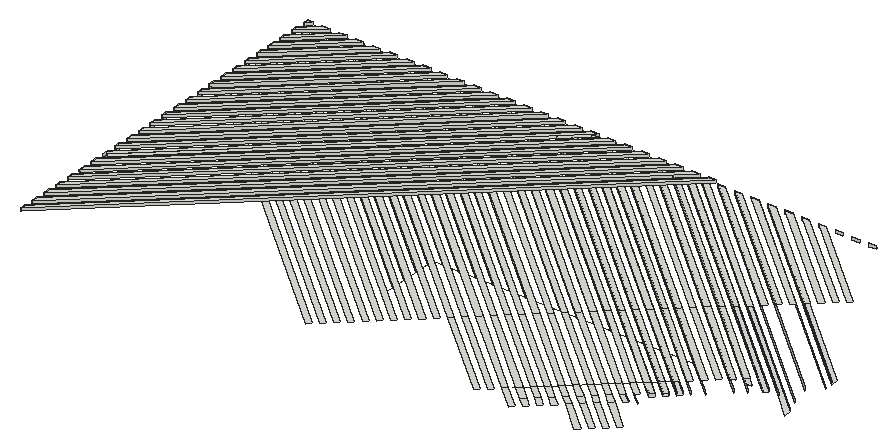
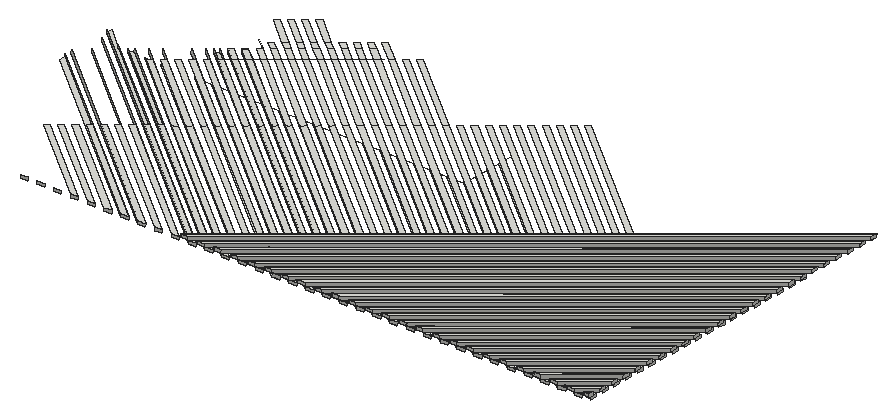
# SketchUp Ruby script. Lengths in inches.
U = 1.inch
M = Sketchup.active_model
def pt(a) = Geom::Point3d.new(a.map { |v| v * U })
def face(e, loops, mat)
  f = e.add_face(loops[0].map { |a| pt(a) })
  loops[1..].each { |l| e.add_face(l.map { |a| pt(a) }).erase! }
  f.material = f.back_material = mat if mat
  f
end
# faces: each face lists its corners as indices into pts; further lists are holes
def faces(e, pts, list, mat = nil) = list.each { |f| face(e, (f[0].is_a?(Array) ? f : [f]).map { |l| l.map { |i| pts[i] } }, mat) }
# xy, xz, yz: faces in a plane at the given z, y or x. An outline is a flat list of corners, or four numbers for a rectangle; further outlines are holes
def ring(l) = l.size == 4 ? [[l[0], l[1]], [l[2], l[1]], [l[2], l[3]], [l[0], l[3]]] : l.each_slice(2).to_a
def flat(e, list, mat, &to3) = list.each { |f| face(e, (f[0].is_a?(Array) ? f : [f]).map { |l| ring(l).map { |u, v| to3.(u, v) } }, mat) }
def xy(e, z, list, mat = nil) = flat(e, list, mat) { |x, y| [x, y, z] }
def xz(e, y, list, mat = nil) = flat(e, list, mat) { |x, z| [x, y, z] }
def yz(e, x, list, mat = nil) = flat(e, list, mat) { |y, z| [x, y, z] }
def lines(e, pts, list) = list.each { |a, b| e.add_line(pt(pts[a]), pt(pts[b])) }
# prism: a flat outline (further loops are holes) pulled along v
def prism(e, loops, v, mat = nil)
  f = face(e, loops, mat); d = Geom::Vector3d.new(v.map { |x| x * U })
  f.pushpull(f.normal.samedirection?(d) ? d.length : -d.length)
end
def box(e, o, s, mat = nil) = prism(e, [[o, [o[0] + s[0], o[1], o[2]], [o[0] + s[0], o[1] + s[1], o[2]], [o[0], o[1] + s[1], o[2]]]], [0, 0, s[2]], mat)
def at(x, y, z, deg = 0) = Geom::Transformation.translation(pt([x, y, z])) * Geom::Transformation.rotation(ORIGIN, Z_AXIS, deg.degrees)
def axes(o, x, y, z) = Geom::Transformation.new([*x, 0, *y, 0, *z, 0, *pt(o).to_a, 1])
def part(name) = M.definitions.add(name)
# library, detail: a bought-in or finely detailed component or shape, given as its bounding box
def library(name, o, s) = part(name).tap { |d| box(d.entities, o, s) }
def detail(e, o, s) = box(e.add_group.entities, o, s)
def put(e, d, t, mat = nil) = e.add_instance(d, t).tap { |i| i.material = mat if mat }
def group(e, t, mat = nil) = e.add_group.tap { |g| g.transformation = t; g.material = mat if mat }.entities
root = M.entities
yz(root,1643.753,[[641.527,112.68,643.815,112.761,643.793,113.788,641.504,113.707]])
yz(root,1643.781,[[646.852,112.869,646.829,113.896,649.182,113.979,649.205,112.952]])
yz(root,1643.818,[[650.825,111.952,650.802,112.979,653.091,113.06,653.113,112.033]])
yz(root,1643.819,[[640.161,111.574,640.139,112.601,642.427,112.682,642.45,111.655],[645.46,111.762,645.437,112.789,647.79,112.872,647.813,111.845]])
yz(root,1643.82,[[624.133,111.006,624.11,112.033,626.463,112.116,626.486,111.089],[629.498,111.196,629.475,112.223,631.764,112.304,631.786,111.277]])
yz(root,1643.821,[[613.469,110.628,613.447,111.655,615.8,111.738,615.822,110.711],[618.834,110.818,618.812,111.845,621.1,111.926,621.123,110.899]])
yz(root,1643.822,[[602.806,110.25,602.783,111.277,605.136,111.36,605.159,110.333],[608.171,110.44,608.148,111.467,610.437,111.548,610.459,110.521]])
yz(root,1643.823,[[586.844,109.684,589.132,109.765,589.11,110.792,586.821,110.711],[592.143,109.872,594.496,109.955,594.473,110.982,592.12,110.899]])
yz(root,1643.824,[[576.181,109.306,578.469,109.387,578.446,110.414,576.158,110.333],[581.479,109.494,583.832,109.577,583.81,110.604,581.456,110.521]])
yz(root,1643.825,[[560.152,108.738,562.505,108.821,562.483,109.848,560.13,109.765],[565.517,108.928,567.806,109.009,567.783,110.036,565.494,109.955]])
yz(root,1643.826,[[554.854,108.55,557.142,108.631,557.119,109.658,554.831,109.577]])
p = [[1824.097,523.211,108.456],[1816.22,530.052,108.698],[1814.866,528.875,108.657],[1822.742,522.034,108.414],[1824.886,573.509,109.211],[1850.385,551.364,108.426],
  [1850.385,551.341,109.453],[1845.556,555.535,109.602],[1814.866,582.188,110.547],[1732.252,653.937,113.09],[1732.252,653.96,112.063],[1851.739,552.54,108.468],
  [1851.739,552.518,109.495],[1827.595,573.509,109.211],[1643.821,613.447,111.655],[1747.351,523.533,108.467],[1748.706,524.71,108.509],[1645.435,614.399,111.689],
  [1645.176,614.623,111.697],[1643.821,615.8,111.738],[1778.04,550.195,109.412],[1808.727,523.543,108.468],[1810.082,524.72,108.509],[1779.394,551.371,109.454],
  [1845.566,523.538,108.467],[1846.92,524.715,108.509],[1836.372,533.876,108.834],[1835.018,532.699,108.792],[1643.135,523.684,108.502],[1643.147,525.983,108.584],
  [1643.137,523.686,108.502],[1643.137,523.663,109.529],[1643.147,525.96,109.611],[1643.151,523.675,109.53],[1643.151,523.697,108.503],[1793.076,653.94,113.12],
  [1793.076,653.917,114.147],[1643.162,525.996,108.584],[1790.442,653.94,113.12],[1825.83,524.717,108.509],[1827.147,525.861,108.55],[1824.1,528.508,108.644],
  [1822.783,527.363,108.603],[1734.961,653.96,112.063],[1734.961,653.937,113.09],[1816.22,583.365,110.588],[1846.91,556.711,109.643],[1831.0625,573.509,109.211],
  [1853.473,554.046,108.521],[1853.473,554.024,109.548],[1848.644,558.217,109.697],[1817.954,584.871,110.642],[1738.428,653.9375,113.09],[1738.428,653.96,112.063],
  [1833.697,573.509,109.211],[1854.79,555.191,108.562],[1643.149,525.962,109.611],[1643.162,525.974,109.611],[1790.442,653.917,114.147],[1643.821,618.812,111.845],
  [1750.439,526.216,108.562],[1751.757,527.36,108.603],[1645.138,619.956,111.886],[1643.821,621.1,111.926],[1781.128,552.877,109.507],[1811.816,526.226,108.5625],
  [1813.133,527.37,108.603],[1782.445,554.022,109.548],[1848.654,526.221,108.5625],[1849.971,527.365,108.603],[1839.423,536.526,108.928],[1838.106,535.382,108.887],
  [1819.271,532.702,108.792],[1817.954,531.558,108.752],[1828.88,527.367,108.603],[1830.234,528.543,108.645],[1827.1875,531.189,108.739],[1825.833,530.013,108.697],
  [1753.929,555.196,108.562],[1643.818,650.825,111.952],[1643.818,653.113,112.033],[1645.136,651.969,111.993],[1649.024,648.592,111.873],[1753.929,557.485,108.643],
  [1741.0625,653.96,112.063],[1741.0625,653.9375,113.09],[1819.271,586.015,110.682],[1849.961,559.362,109.737],[1854.79,555.168,109.589],[1837.162,573.51,109.211],
  [1856.523,556.696,108.615],[1856.523,556.673,109.642],[1851.694,560.867,109.791],[1821.004,587.521,110.736],[1744.528,653.938,113.09],[1744.528,653.96,112.063],
  [1839.871,573.51,109.211],[1857.877,557.872,108.657],[1643.82,624.11,112.033],[1753.489,528.866,108.656],[1754.844,530.042,108.698],[1648.824,622.117,111.962],
  [1645.175,625.287,112.075],[1643.82,626.463,112.116],[1784.178,555.527,109.601],[1785.532,556.704,109.643],[1842.51,539.208,109.023],[1841.155,538.031,108.981],
  [1851.703,528.871,108.656],[1853.057,530.048,108.698],[1643.162,529.008,108.691],[1643.175,531.372,108.775],[1643.165,529.011,108.691],[1643.165,528.988,109.718],
  [1643.175,531.349,109.802],[1643.19,531.385,108.775],[1643.178,529.022,108.691],[1786.974,653.94,113.12],[1784.265,653.94,113.12],[1643.178,528.999,109.718],
  [1786.974,653.917,114.147],[1822.358,535.384,108.887],[1821.004,534.207,108.846],[1831.968,530.049,108.698],[1833.285,531.194,108.739],[1830.238,533.84,108.833],
  [1828.921,532.695,108.792],[1747.237,653.961,112.063],[1747.237,653.938,113.09],[1822.358,588.697,110.777],[1853.048,562.043,109.832],[1857.877,557.85,109.684],
  [1843.339,573.51,109.211],[1859.611,559.379,108.71],[1859.611,559.356,109.737],[1854.782,563.549,109.886],[1824.092,590.203,110.831],[1750.705,653.938,113.09],
  [1750.705,653.961,112.063],[1650.66,650.181,111.929],[1646.315,653.955,112.063],[1649.024,653.955,112.063],[1753.928,562.848,108.833],[1753.928,560.495,108.75],
  [1643.177,531.352,109.802],[1643.19,531.363,109.802],[1784.265,653.917,114.147],[1643.82,629.475,112.223],[1756.577,531.548,108.751],[1757.894,532.693,108.792],
  [1645.849,630.001,112.242],[1645.137,630.619,112.264],[1643.82,631.764,112.304],[1787.266,558.21,109.697],[1788.583,559.354,109.737],[1845.561,541.858,109.117],
  [1844.243,540.714,109.076],[1854.791,531.554,108.752],[1856.108,532.698,108.792],[1825.409,538.034,108.981],[1824.092,536.89,108.941],[1833.325,536.522,108.928],
  [1831.971,535.345,108.886],[1643.82,634.774,112.411],[1759.627,534.198,108.845],[1760.981,535.374,108.887],[1648.863,632.746,112.339],[1645.174,635.95,112.453],
  [1643.819,637.127,112.494],[1790.315,560.859,109.79],[1791.67,562.036,109.832],[1849.439,573.51,109.211],[1862.66,562.028,108.804],[1862.66,562.005,109.831],
  [1857.832,566.199,109.98],[1827.141,592.853,110.925],[1756.805,653.939,113.09],[1756.805,653.961,112.063],[1643.19,534.396,108.882],[1643.202,536.695,108.963],
  [1643.193,534.399,108.882],[1643.217,536.708,108.964],[1643.205,534.409,108.882],[1780.8,653.939,113.12],[1778.165,653.939,113.12],[1643.193,534.376,109.909],
  [1643.202,536.672,109.99],[1643.205,534.386,109.909],[1780.8,653.917,114.147],[1828.496,540.716,109.076],[1827.142,539.539,109.035],[1836.376,539.172,109.022],
  [1835.059,538.028,108.981],[1643.819,640.139,112.601],[1762.715,536.881,108.94],[1764.032,538.025,108.981],[1648.646,638.235,112.534],[1645.905,640.615,112.618],
  [1645.136,641.283,112.642],[1643.819,642.427,112.682],[1793.403,563.542,109.886],[1794.72,564.686,109.926],[1656.638,650.354,111.936],[1652.491,653.955,112.063],
  [1655.126,653.955,112.063],[1753.928,568.148,109.021],[1753.928,565.86,108.94],[1643.205,536.675,109.99],[1643.217,536.685,109.991],[1778.165,653.917,114.147],
  [1831.547,543.366,109.17],[1830.23,542.222,109.13],[1839.463,541.854,109.117],[1838.109,540.677,109.075],[1643.819,645.437,112.789],[1765.765,539.53,109.034],
  [1767.119,540.707,109.076],[1648.501,643.723,112.728],[1645.173,646.614,112.831],[1643.819,647.79,112.872],[1796.453,566.191,109.98],[1797.807,567.368,110.021],
  [1790.169,653.963,112.064],[1888.287,568.751,109.043],[1888.287,566.462,108.961],[1880.169,573.512,109.211],[1787.535,653.963,112.064],[1861.716,573.511,109.211],
  [1868.798,567.36,108.993],[1868.798,567.337,110.02],[1863.97,571.531,110.169],[1833.279,598.185,111.114],[1769.081,653.939,113.09],[1769.081,653.962,112.063],
  [1843.822,607.345,111.438],[1882.387,573.852,110.251],[1888.287,568.728,110.069],[1790.169,653.941,113.09],[1643.218,539.72,109.071],[1643.23,542.084,109.155],
  [1643.221,539.723,109.071],[1643.245,542.097,109.155],[1643.233,539.733,109.071],[1643.221,539.701,110.098],[1643.23,542.062,110.181],[1643.233,539.711,110.098],
  [1774.697,653.939,113.12],[1774.697,653.916,114.147],[1771.988,653.939,113.12],[1834.634,546.048,109.265],[1833.28,544.871,109.224],[1842.514,544.504,109.211],
  [1841.197,543.36,109.17],[1647.158,647.902,112.876],[1768.852,542.213,109.129],[1770.17,543.357,109.17],[1648.693,648.857,112.91],[1645.136,651.946,113.02],
  [1643.818,653.091,113.06],[1643.818,650.802,112.979],[1799.541,568.874,110.075],[1800.858,570.019,110.115],[1867.892,573.512,109.211],[1871.886,570.043,109.088],
  [1871.886,570.02,110.115],[1867.058,574.213,110.264],[1836.367,600.868,111.209],[1775.258,653.94,113.09],[1775.258,653.962,112.063],[1643.824,573.146,110.226],
  [1643.825,570.793,110.143],[1643.825,570.816,109.116],[1643.824,573.169,109.199],[1666.086,647.447,111.832],[1658.592,653.955,112.063],[1661.301,653.955,112.063],
  [1753.935,573.505,109.211],[1753.927,573.505,109.211],[1753.927,571.158,109.128],[1643.233,542.065,110.182],[1643.245,542.074,110.182],[1771.988,653.916,114.147],
  [1837.685,548.698,109.359],[1836.368,547.554,109.319],[1847.293,543.363,109.17],[1848.646,544.539,109.212],[1845.601,547.186,109.306],[1844.247,546.009,109.264],
  [1848.647,544.54,109.212],[1650.696,650.127,112.955],[1771.902,544.862,109.223],[1773.257,546.039,109.265],[1649.024,653.932,113.09],[1646.315,653.932,113.09],
  [1802.591,571.524,110.169],[1803.945,572.7,110.21],[1873.992,573.512,109.211],[1874.936,572.692,109.182],[1874.936,572.67,110.209],[1870.108,576.863,110.358],
  [1839.417,603.517,111.303],[1781.358,653.94,113.09],[1781.358,653.963,112.064],[1784.067,653.963,112.064],[1876.291,573.869,109.224],[1875.88,573.512,109.211],
  [1672.223,647.481,111.834],[1664.768,653.956,112.063],[1667.403,653.956,112.063],[1760.037,573.505,109.211],[1757.402,573.505,109.211],[1675.176,650.215,111.931],
  [1670.868,653.956,112.063],[1673.577,653.956,112.063],[1766.212,573.505,109.211],[1763.503,573.505,109.211],[1681.352,650.216,111.931],[1677.045,653.956,112.063],
  [1679.679,653.957,112.063],[1772.314,573.506,109.211],[1769.679,573.506,109.211],[1688.123,649.634,111.91],[1683.145,653.957,112.063],[1685.854,653.957,112.063],
  [1778.488,573.506,109.211],[1775.779,573.506,109.211],[1694.299,649.634,111.91],[1689.321,653.957,112.063],[1691.956,653.957,112.063],[1784.59,573.507,109.211],
  [1781.956,573.506,109.211],[1700.724,649.352,111.9],[1695.422,653.958,112.063],[1698.131,653.958,112.063],[1790.765,573.507,109.211],[1788.056,573.507,109.211],
  [1806.509,573.508,109.211],[1713.875,653.959,112.063],[1716.509,653.959,112.063],[1809.144,573.508,109.211],[1812.609,573.508,109.211],[1719.975,653.959,112.063],
  [1722.684,653.959,112.063],[1815.318,573.508,109.211],[1818.786,573.509,109.211],[1726.151,653.959,112.063],[1728.786,653.959,112.063],[1821.42,573.509,109.211],
  [1753.339,653.961,112.063],[1845.974,573.51,109.211],[1759.514,653.961,112.063],[1852.148,573.511,109.211],[1771.79,653.962,112.063],[1864.425,573.511,109.211],
  [1777.893,653.962,112.063],[1870.527,573.512,109.211],[1880.169,573.49,110.238],[1842.505,606.2,111.398],[1787.535,653.94,113.09],[1793.635,653.963,112.064],
  [1886.269,573.513,109.211],[1886.269,573.49,110.238],[1884.119,575.357,110.304],[1845.554,608.85,111.492],[1793.635,653.941,113.09],[1784.067,653.94,113.09],
  [1840.771,604.694,111.345],[1871.463,578.039,110.4],[1876.291,573.846,110.251],[1848.608,547.519,109.347],[1851.662,544.872,109.253],[1851.658,544.868,109.253],
  [1848.607,547.518,109.347],[1653.992,554.422,110.62],[1643.26,545.098,110.289],[1643.249,545.089,110.289],[1643.249,545.111,109.262],[1643.26,545.121,109.262],
  [1649.213,550.292,109.446],[1768.523,653.939,113.12],[1768.523,653.916,114.147],[1643.257,547.384,110.37],[1643.257,547.407,109.343],[1643.272,547.42,109.344],
  [1647.895,551.436,109.486],[1840.772,551.379,109.454],[1839.418,550.203,109.413],[1649.742,553.04,109.543],[1643.261,547.388,110.37],[1643.272,547.397,110.371],
  [1652.935,555.791,110.668],[1765.888,653.916,114.147],[1765.888,653.938,113.12],[1656.638,650.331,112.962],[1774.99,547.545,109.318],[1776.307,548.689,109.359],
  [1655.126,653.933,113.09],[1652.491,653.932,113.09],[1847.252,548.695,109.389],[1805.679,574.206,110.264],[1806.996,575.351,110.304],[1848.652,549.836,109.4],
  [1843.823,554.03,109.548],[1842.506,552.885,109.508],[1847.335,548.692,109.359],[1665.424,647.999,112.88],[1661.301,653.933,113.09],[1658.592,653.933,113.09],
  [1808.728,576.856,110.358],[1810.083,578.033,110.399],[1648.834,555.241,110.649],[1643.287,550.422,110.478],[1643.277,550.414,110.478],[1643.277,550.436,109.451],
  [1643.287,550.445,109.451],[1646.161,552.942,109.539],[1650.485,556.698,109.673],[1762.421,653.938,113.12],[1762.421,653.916,114.147],[1643.273,550.432,109.451],
  [1643.285,552.796,109.534],[1643.299,552.809,109.535],[1643.285,552.774,110.561],[1644.807,554.118,109.581],[1646.715,555.776,109.64],[1643.289,552.778,110.561],
  [1643.299,552.786,110.562],[1646.387,555.469,110.657],[1759.712,653.915,114.147],[1759.712,653.938,113.12],[1671.6,648,112.88],[1667.403,653.933,113.09],
  [1664.768,653.933,113.09],[1811.816,579.539,110.453],[1813.133,580.683,110.493],[1881.944,582.633,109.535],[1884.162,580.707,109.466],[1884.162,580.684,110.493],
  [1848.642,611.532,111.587],[1799.811,653.941,113.09],[1799.811,653.964,112.064],[1675.176,650.193,112.958],[1673.577,653.934,113.09],[1670.868,653.933,113.09],
  [1643.3,555.82,109.642],[1643.312,558.119,109.723],[1643.305,555.824,109.642],[1643.326,558.131,109.723],[1643.315,555.832,109.642],[1756.246,653.915,114.147],
  [1643.315,555.81,110.669],[1643.305,555.802,110.669],[1756.246,653.938,113.12],[1643.312,558.096,110.75],[1753.612,653.938,113.12],[1853.046,615.359,111.723],
  [1888.285,584.754,110.638],[1888.285,584.777,109.611],[1808.62,653.964,112.064],[1808.62,653.942,113.09],[1643.317,558.101,110.75],[1643.326,558.109,110.75],
  [1753.612,653.915,114.147],[1683.983,647.908,112.877],[1679.679,653.934,113.09],[1677.045,653.934,113.09],[1888.285,587.789,109.717],[1812.088,653.964,112.064],
  [1814.723,653.965,112.064],[1888.285,590.077,109.799],[1888.285,587.766,110.744],[1854.78,616.865,111.776],[1812.088,653.942,113.09],[1690.639,647.425,112.859],
  [1685.854,653.934,113.09],[1683.145,653.934,113.09],[1643.34,563.508,109.914],[1643.345,563.513,109.914],[1643.328,561.144,109.83],[1643.345,563.49,110.941],
  [1643.328,561.122,110.857],[1643.354,563.52,109.915],[1643.342,561.157,109.831],[1750.144,653.9375,113.12],[1747.435,653.9375,113.12],[1747.435,653.915,114.147],
  [1643.354,563.498,110.941],[1693.825,650.023,112.952],[1691.956,653.935,113.09],[1689.321,653.935,113.09],[1856.099,564.694,109.926],[1825.409,591.348,110.871],
  [1699.728,650.195,112.958],[1698.131,653.935,113.09],[1695.422,653.935,113.09],[1859.187,567.375,110.021],[1828.496,594.03,110.966],[1643.355,566.532,110.021],
  [1643.367,568.831,110.103],[1643.361,566.537,110.021],[1643.381,568.843,110.103],[1643.369,566.544,110.022],[1743.97,653.937,113.12],[1741.335,653.937,113.12],
  [1643.369,566.522,111.049],[1643.361,566.514,111.048],[1743.97,653.915,114.147],[1643.367,568.808,111.13],[1643.373,568.813,111.13],[1643.381,568.82,111.13],
  [1741.335,653.914,114.147],[1705.637,650.428,112.966],[1704.233,653.935,113.09],[1701.598,653.935,113.09],[1830.229,595.536,111.02],[1860.92,568.881,110.075],
  [1862.237,570.026,110.115],[1831.547,596.68,111.06],[1643.823,597.485,111.089],[1643.822,599.773,111.17],[1643.822,599.796,110.143],[1643.823,597.507,110.062],
  [1707.698,653.936,113.09],[1710.407,653.936,113.09],[1865.325,572.707,110.211],[1834.633,599.362,111.155],[1643.397,571.846,111.237],[1643.389,571.839,111.237],
  [1643.389,571.862,110.21],[1643.397,571.868,110.21],[1737.867,653.937,113.12],[1737.867,653.914,114.147],[1643.395,574.198,111.321],[1643.395,574.22,110.294],
  [1643.383,571.857,110.21],[1643.409,574.232,110.294],[1735.158,653.937,113.12],[1643.822,602.806,110.25],[1643.822,605.159,110.333],[1645.177,603.983,110.292],
  [1643.401,574.203,111.321],[1643.409,574.21,111.321],[1735.158,653.914,114.147],[1713.875,653.936,113.09],[1716.509,653.936,113.09],[1868.376,575.358,110.304],
  [1837.684,602.012,111.249],[1643.822,605.136,111.36],[1645.177,603.96,111.319],[1719.975,653.936,113.09],[1722.684,653.937,113.09],[1643.411,577.244,110.401],
  [1643.422,579.543,110.483],[1643.417,577.25,110.401],[1643.424,577.233,111.428],[1643.417,577.227,111.428],[1643.424,577.256,110.401],[1731.693,653.936,113.12],
  [1731.693,653.914,114.147],[1643.422,579.52,111.509],[1643.436,579.555,110.483],[1729.058,653.936,113.12],[1643.822,608.171,110.44],[1643.822,610.459,110.521],
  [1645.139,609.315,110.481],[1643.429,579.526,111.51],[1643.436,579.532,111.51],[1729.058,653.914,114.147],[1726.151,653.937,113.09],[1728.786,653.937,113.09],
  [1643.822,610.437,111.548],[1645.139,609.293,111.508],[1643.438,582.569,110.59],[1643.45,584.932,110.674],[1643.445,582.575,110.59],[1643.451,582.558,111.617],
  [1643.445,582.552,111.617],[1643.451,582.58,110.59],[1725.591,653.936,113.12],[1725.591,653.913,114.147],[1643.45,584.91,111.701],[1643.463,584.944,110.674],
  [1722.882,653.936,113.12],[1643.821,613.469,110.628],[1643.821,615.822,110.711],[1645.176,614.646,110.67],[1643.457,584.916,111.701],[1643.463,584.921,111.701],
  [1722.882,653.913,114.147],[1643.479,587.945,111.808],[1643.473,587.94,111.808],[1643.473,587.963,110.781],[1643.479,587.968,110.781],[1719.416,653.936,113.12],
  [1719.416,653.913,114.147],[1643.478,590.232,111.889],[1643.478,590.255,110.862],[1643.466,587.956,110.781],[1643.491,590.266,110.863],[1716.782,653.936,113.12],
  [1753.339,653.938,113.09],[1643.821,618.834,110.818],[1643.821,621.123,110.899],[1645.138,619.979,110.859],[1643.333,561.126,110.857],[1643.342,561.134,110.858],
  [1750.144,653.915,114.147],[1643.485,590.239,111.889],[1643.491,590.244,111.89],[1716.782,653.913,114.147],[1759.514,653.939,113.09],[1705.723,647.341,112.886],
  [1643.506,593.292,110.97],[1643.518,595.656,111.054],[1702.045,646.499,112.856],[1704.368,648.517,112.928],[1643.505,595.622,112.08],[1643.505,595.644,111.053],
  [1643.501,593.288,110.97],[1643.501,593.265,111.997],[1643.506,593.269,111.997],[1713.314,653.935,113.12],[1713.314,653.913,114.147],[1701.477,643.63,113.782],
  [1643.493,593.281,110.97],[1762.981,653.939,113.09],[1765.616,653.939,113.09],[1643.82,624.133,111.006],[1643.82,626.486,111.089],[1645.175,625.309,111.048],
  [1643.513,595.629,112.081],[1643.518,595.633,112.081],[1710.605,653.913,114.147],[1710.605,653.935,113.12],[1771.79,653.939,113.09],[1643.533,598.657,112.188],
  [1643.529,598.653,112.188],[1643.529,598.676,111.161],[1643.533,598.679,111.161],[1707.14,653.935,113.12],[1707.14,653.912,114.147],[1703.361,650.63,114.03],
  [1643.533,600.967,111.242],[1643.545,600.978,111.242],[1643.533,600.945,112.269],[1704.505,653.935,113.12],[1643.541,600.952,112.269],[1643.545,600.955,112.269],
  [1704.505,653.912,114.147],[1777.893,653.94,113.09],[1643.82,629.498,111.196],[1643.82,631.786,111.277],[1645.137,630.642,111.237],[1643.548,603.993,111.349],
  [1643.56,606.357,111.433],[1643.557,604,111.35],[1643.561,603.981,112.377],[1643.557,603.978,112.377],[1643.561,604.004,111.35],[1701.038,653.935,113.12],
  [1701.038,653.912,114.147],[1643.573,606.367,111.434],[1698.329,653.934,113.12],[1643.56,606.334,112.46],[1643.569,606.342,112.46],[1643.573,606.345,112.46],
  [1698.329,653.912,114.147],[1643.819,637.149,111.467],[1643.82,634.796,111.384],[1645.174,635.973,111.426],[1846.909,610.026,111.534],[1796.344,653.941,113.09],
  [1694.863,653.934,113.12],[1643.588,609.391,111.541],[1643.6,611.69,111.622],[1692.228,653.934,113.12],[1643.576,609.38,111.54],[1643.588,611.679,111.622],
  [1643.585,609.388,111.541],[1694.863,653.912,114.147],[1643.588,609.368,112.568],[1643.585,609.366,112.568],[1643.588,611.657,112.649],[1849.96,612.677,111.628],
  [1802.446,653.941,113.09],[1643.597,611.665,112.649],[1643.6,611.667,112.649],[1692.228,653.911,114.147],[1643.819,640.161,111.574],[1643.819,642.45,111.655],
  [1645.136,641.306,111.615],[1805.911,653.941,113.09],[1851.692,614.182,111.681],[1643.603,614.705,111.729],[1643.616,617.069,111.813],[1643.613,614.713,111.729],
  [1643.613,614.691,112.756],[1643.616,617.046,112.84],[1688.761,653.934,113.12],[1643.615,614.715,111.729],[1643.627,617.079,111.813],[1686.052,653.934,113.12],
  [1643.615,614.693,112.756],[1688.761,653.911,114.147],[1856.097,618.009,111.817],[1814.723,653.942,113.09],[1643.625,617.055,112.84],[1643.627,617.056,112.84],
  [1686.052,653.911,114.147],[1645.173,646.636,111.804],[1643.819,647.813,111.845],[1818.188,653.942,113.091],[1857.83,619.514,111.87],[1859.184,620.691,111.912],
  [1820.897,653.942,113.091],[1643.641,620.079,112.947],[1643.641,620.101,111.92],[1643.643,622.391,112.002],[1643.643,622.369,113.029],[1643.643,620.08,112.947],
  [1643.643,620.103,111.92],[1682.586,653.933,113.12],[1682.586,653.911,114.147],[1643.655,622.401,112.002],[1679.952,653.933,113.12],[1643.631,620.092,111.92],
  [1824.365,653.943,113.091],[1860.918,622.197,111.965],[1862.235,623.341,112.006],[1826.999,653.943,113.091],[1643.653,622.378,113.029],[1643.655,622.379,113.029],
  [1679.952,653.911,114.147],[1830.465,653.943,113.091],[1863.967,624.847,112.059],[1865.322,626.023,112.101],[1833.174,653.943,113.091],[1643.669,625.403,113.136],
  [1643.671,627.758,113.22],[1643.671,627.781,112.193],[1643.669,625.426,112.109],[1643.67,625.404,113.136],[1643.67,625.427,112.109],[1676.484,653.933,113.12],
  [1676.484,653.911,114.147],[1643.682,627.791,112.193],[1673.775,653.933,113.12],[1643.658,625.417,112.109],[1701.598,653.958,112.063],[1704.233,653.958,112.063],
  [1710.407,653.958,112.063],[1707.698,653.958,112.063],[1765.616,653.962,112.063],[1762.981,653.962,112.063],[1796.344,653.964,112.064],[1802.446,653.964,112.064],
  [1805.911,653.964,112.064],[1820.897,653.965,112.064],[1818.188,653.965,112.064],[1826.999,653.965,112.064],[1824.365,653.965,112.064],[1833.174,653.966,112.064],
  [1830.465,653.966,112.064],[1836.641,653.943,113.091],[1839.276,653.943,113.091],[1839.276,653.966,112.064],[1836.641,653.966,112.064],[1842.741,653.944,113.091],
  [1845.45,653.944,113.091],[1845.45,653.966,112.064],[1842.741,653.966,112.064],[1848.918,653.944,113.091],[1851.553,653.944,113.091],[1851.553,653.967,112.064],
  [1848.918,653.967,112.064],[1643.681,627.767,113.22],[1673.775,653.91,114.147],[1670.31,653.91,114.147],[1643.697,630.791,113.327],[1643.697,630.814,112.3],
  [1670.31,653.933,113.12],[1643.709,633.113,112.382],[1667.675,653.933,113.12],[1643.698,633.103,112.381],[1643.698,633.081,113.408],[1643.686,630.804,112.3],
  [1643.709,633.09,113.409],[1667.675,653.91,114.147],[1643.714,636.129,112.489],[1643.726,638.493,112.572],[1643.725,636.139,112.489],[1643.725,636.116,113.516],
  [1643.725,638.47,113.599],[1664.208,653.932,113.12],[1661.499,653.932,113.12],[1664.208,653.91,114.147],[1643.737,638.48,113.6],[1661.499,653.91,114.147],
  [1643.741,641.517,112.68],[1643.753,643.815,112.761],[1643.753,641.527,112.68],[1658.033,653.909,114.147],[1643.753,641.504,113.707],[1658.033,653.932,113.12],
  [1655.398,653.932,113.12],[1643.753,643.793,113.788],[1643.765,643.803,113.788],[1655.398,653.909,114.147],[1651.931,653.909,114.147],[1643.781,646.829,113.896],
  [1643.781,646.852,112.869],[1651.931,653.932,113.12],[1643.781,649.205,112.952],[1649.222,653.931,113.12],[1649.222,653.909,114.147],[1643.781,649.182,113.979],
  [1643.793,649.193,113.98],[1643.809,652.24,113.03],[1643.809,652.24,113.06],[1643.809,652.217,114.087],[1643.818,653.909,114.147],[1643.818,653.931,113.12],
  [1643.818,653.932,113.09],[1645.756,653.909,114.147],[1644.303,652.669,113.075],[1645.756,653.931,113.12],[1643.818,652.669,113.075],[1753.929,552.184,108.455],
  [1794.232,573.507,109.211],[1800.333,573.507,109.211],[1803.042,573.508,109.211],[1796.867,573.507,109.211],[1817.087,530.805,108.725],[1643.521,598.668,111.161]]
faces(root,p,[[0,1,2,3],[4,5,6,7,8,9,10],[5,11,12,6],[5,4,13,11],[14,15,16,17,18,19],[20,21,22,23],[24,25,26,27],[28,29,30],
  [31,32,29,30],[33,31,30,34,35,36],[29,37,34,30],[35,34,37,38],[39,40,41,42],[13,43,44,45,46,12,11],[47,48,49,50,51,52,53],[48,47,54,55],
  [37,29,32,56,57,58,38],[59,60,61,62,63],[64,65,66,67],[68,69,70,71],[41,72,73,42],[74,75,76,77],[78,79,80,81,82,83],[54,84,85,86,87,88,55],
  [89,90,91,92,93,94,95],[90,89,96,97],[98,99,100,101,102,103],[104,2,1,105],[106,107,108,109],[110,111,112],[111,112,113,114],[111,115,116,112],
  [117,116,115,118],[119,113,112,116,117,120],[76,121,122,77],[123,124,125,126],[96,127,128,129,130,131,97],[132,133,134,135,136,137,138],[139,140,141,142,143],[115,111,114,144,145,146,118],
  [147,148,149,150,151,152],[153,73,72,154],[155,156,157,158],[125,159,160,126],[27,26,161,162],[163,164,165,166,167,168],[169,122,121,170],[171,172,173,174,175,176,177],
  [178,179,180],[179,181,182,180],[183,182,181,184],[179,180,185,186],[187,185,180,182,183,188],[161,189,190,162],[71,70,191,192],[193,194,195,196,197,198,199],
  [200,160,159,201],[202,203,204,205,206],[181,179,186,207,208,209,184],[191,210,211,192],[212,213,107,106],[214,215,216,217,218,219],[220,190,189,221],[222,223,224,225,226],
  [227,228,229,230,231,232,233],[234,235,236,223,222,237],[238,239,240],[239,241,242,240],[239,240,243,244],[245,243,240,242,246,247],[246,242,241,248],[212,249,250,213],
  [251,252,156,155],[253,254,255,256,257,258,259],[260,211,210,261],[262,263,264,265,266,267,268],[269,270,271,272],[273,274,275,276,277,278],[241,239,244,279,280,281,248],[251,282,283,252],
  [284,285,286,287],[288,286,285],[289,290,291,292,293],[294,250,249,295],[296,297,298,299,300,301,302],[297,296,302,303,304,305],[306,307,308,309,310],[311,312,313,314,315],
  [316,317,318,319,320],[321,322,323,324,325],[326,327,328,329,330],[331,332,333,334,335],[336,337,338,339],[340,341,342,343],[344,345,346,347],[4,10,43,13],
  [47,53,84,54],[89,95,127,96],[132,138,348,349],[171,177,350,351],[227,233,352,353],[262,268,354,355],[226,225,356,357,358],[359,360,361,362,363,364],
  [304,303,365,366,367,368],[369,370,371,372],[373,374,375,376,377,378,379,380],[376,375,381,382],[382,383,377,376],[378,377,383,384],[286,385,386,287],[387,384,383,382,381,388,389,390,391,392],
  [393,394,395,396,397],[372,398,369],[399,283,282,400],[401,402,403,404],[405,20,23,406,407],[408,386,385,409],[384,387,392,379,378],[57,56,31,33,36,58],
  [56,32,31],[410,411,412,413,414,415,416,417,418],[419,420,413],[420,421,414,413],[422,420,413,412],[415,414,421,423],[12,46,7,6],[424,423,421,420,422,425,426,427,428,429],
  [423,424,429,417,416,415],[430,64,67,431,432],[433,403,402,434],[88,87,50,49],[435,436,437,438,439,440],[441,104,105,442,443],[8,7,46,45],[444,445,446],
  [445,447,448,446],[449,450,451,446,448,452],[451,446,445,453],[452,448,447,454],[455,456,457,458,459],[145,144,113,119,120,146],[144,114,113],[447,445,453,460,461,462,454],
  [463,153,154,464,465],[51,50,87,86],[466,467,468,469],[467,466,470,471,472],[473,169,170,474,475],[93,92,130,129],[476,477,478],[478,477,479,480],
  [477,481,482,478],[483,482,481,484],[208,207,185,187,188,209],[207,186,185],[479,477,481,484,485,486],[487,200,201,488,489],[136,135,490,491],[492,220,221,493,494],
  [175,174,495,496],[497,498,499],[498,500,501,499],[502,501,500,503],[504,505,499,501,502,506],[507,498,499,505],[279,243,245,247,281,280],[279,244,243],
  [500,498,507,508,509,510,503],[511,260,261,512,513],[514,515,516,517],[518,519,520,521],[522,294,295,523],[231,230,524,525],[526,527,528,529,530,531],[532,527,528,533],
  [534,533,528],[530,529,535,536],[533,535,529,528],[537,538,539],[390,389,388,375,374,373,380,391],[388,381,375],[535,533,532,540,541,542,536],[543,399,400,544],
  [266,265,545,546],[538,547,548,539],[549,408,409,550],[551,552,553],[554,555,553,556,557,558],[555,559,552,553],[552,560,556,553],[557,556,560,561],
  [562,563,564],[427,426,425,412,411,410,418,428],[425,422,412],[560,552,559,565,566,567,561],[568,433,434,569],[9,8,45,44],[563,570,571,564],[572,573,574],
  [575,576,574,577,578,579],[573,574,576,580],[573,581,577,574],[578,577,581,582],[52,51,86,85],[583,584,585],[460,451,450,449,462,461],[460,453,451],
  [581,573,580,586,587,588,582],[94,93,129,128],[584,19,18,585],[589,590,591,592,593,594],[595,596,591,590],[597,596,591],[593,592,598,599],[596,598,592,591],
  [137,136,491,600],[601,602,603],[479,604,605,606,485,486],[598,596,595,607,608,609,599],[176,175,496,610],[602,63,62,603],[508,505,504,506,510,509],[508,507,505],
  [611,612,613,614,615],[616,617,618,619],[620,619,618,612,611,621,622,623],[624,617,618],[617,613,612,618],[625,514,517,626],[627,628,629],[628,103,102,629],
  [613,617,616,630,631,632,633,615,614],[232,231,525,634],[540,532,527],[541,540,527,526,531,542],[635,636,637,638,639,640,641],[637,642,643,638],[642,637,636,644],[638,643,645,639],
  [643,642,644,646,647,648,645],[267,266,546,649],[650,651,652],[152,151,652,651],[301,300,366,365],[653,654,655],[656,657,655,658,659,660],[659,658,661,662],
  [663,654,655,657],[654,661,658,655],[565,559,555],[566,565,555,554,558,567],[358,357,234,237],[661,654,663,664,665,666,662],[667,668,163,168],[668,667,669],
  [168,167,669,667],[364,363,670,671],[672,673,674,675],[676,677,678],[677,674,673,678],[679,680,681,678,673,672],[681,682,677,678],[586,580,576],
  [587,586,576,575,579,588],[439,438,683,684],[674,677,682,685,686,687,675],[688,689,690],[199,198,690,689],[691,692,455,459],[693,694,695],[696,697,694,695],
  [698,699,700,701],[702,696,695,699,698,703],[694,700,699,695],[607,595,590],[608,607,590,589,594,609],[472,471,704,705],[700,694,697,706,707,708,701],[219,218,709,710],
  [711,712,713,714],[715,716,717,718],[719,715,716,720,721,722],[721,720,723,724],[725,717,716],[717,723,720,716],[393,397,203,202],[630,616,619],
  [631,630,619,620,623,622,632],[726,727,728,729],[723,717,718,730,731,732,724],[80,258,257,81],[733,734,735,736],[737,738,739,740],[741,737,740,742,743,744],[743,742,745,746],
  [739,745,742,740],[747,739,740],[141,140,293,292],[397,396,204,203],[274,407,406,275],[431,308,307,432],[443,442,313,312],[465,464,318,317],
  [475,474,323,322],[489,488,328,327],[494,493,333,332],[748,513,512,749],[522,523,750,751],[543,544,338,337],[549,550,342,341],[568,569,346,345],
  [9,44,43,10],[52,85,84,53],[94,128,127,95],[137,600,348,138],[176,610,350,177],[625,626,752,753],[232,634,352,233],[267,649,354,268],
  [301,365,303,302],[358,237,222,226],[364,671,754,359],[439,684,755,440],[691,459,458,756],[472,705,468,467],[711,714,757,758],[726,729,759,760],
  [733,736,761,762],[763,764,765,766],[767,768,769,770],[771,772,773,774],[647,646,636,635,641,640,648],[644,636,646],[745,739,738,775,776,746],[777,778,779,780],
  [780,779,781,782],[783,781,779],[778,784,783,779],[785,783,779],[778,786,781,779],[664,663,657],[665,664,657,656,660,666],[782,781,786,787],
  [784,786,781,783],[788,789,790],[790,791,792,789],[793,790,789,794],[795,791,790,793],[685,682,681],[686,685,681,680,679,687],[794,789,792,796,797],
  [798,799,800],[801,802,800,803],[803,800,799,804],[706,697,696],[707,706,696,702,703,708],[804,799,805,806,807],[730,718,715],[731,730,715,719,722,732],
  [808,809,810,811],[811,810,812,813],[621,611,615,633],[814,813,812,815,816],[817,818,819,820,821,822],[775,738,737,741],[776,775,741,744],[823,819,818,824,825],
  [825,824,826,821],[825,821,820,823],[814,808,811,813],[807,801,803,804],[797,795,793,794],[787,777,780,782],[776,744,743,746],[732,722,721,724],
  [708,703,698,701],[687,679,672,675],[666,660,659,662],[645,648,640,639],[632,622,621,633],[609,594,593,599],[588,579,578,582],[567,558,557,561],
  [542,531,530,536],[510,506,502,503],[485,606,483,484],[462,449,452,454],[428,418,417,429],[391,380,379,392],[281,247,246,248],[209,188,183,184],
  [146,120,117,118],[58,36,35,38],[787,786,778,777],[786,784,778],[797,796,791,795],[796,792,791],[807,806,802,801],[806,805,802],
  [816,815,809],[814,816,809,808],[823,820,819]])
lines(root,p,[[320,314],[78,827],[206,142],[335,329],[4,347],[344,343],[132,96],[143,83],[330,324],[315,309],[828,334],[89,54],
  [171,349],[310,276],[160,121],[325,319],[829,751],[278,205],[47,13],[336,830],[829,831],[340,339],[386,282],[73,832],
  [211,189],[92,87],[250,210],[50,46],[403,385],[283,249],[833,637],[122,72],[190,159],[7,402]])
